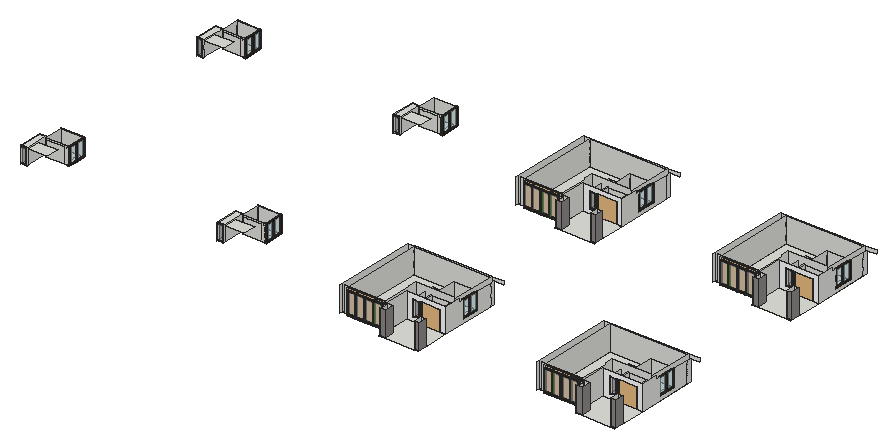
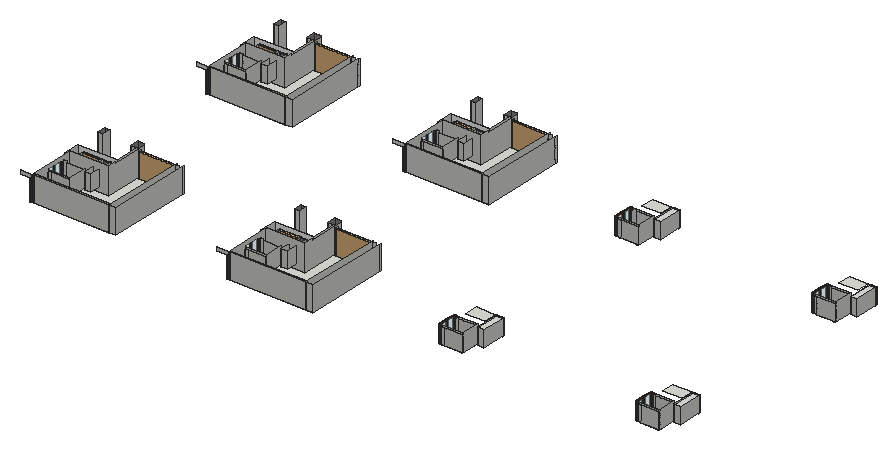
# SketchUp Ruby script. Lengths in inches.
U = 1.inch
M = Sketchup.active_model
def pt(a) = Geom::Point3d.new(a.map { |v| v * U })
def face(e, loops, mat)
  f = e.add_face(loops[0].map { |a| pt(a) })
  loops[1..].each { |l| e.add_face(l.map { |a| pt(a) }).erase! }
  f.material = f.back_material = mat if mat
  f
end
# faces: each face lists its corners as indices into pts; further lists are holes
def faces(e, pts, list, mat = nil) = list.each { |f| face(e, (f[0].is_a?(Array) ? f : [f]).map { |l| l.map { |i| pts[i] } }, mat) }
# xy, xz, yz: faces in a plane at the given z, y or x. An outline is a flat list of corners, or four numbers for a rectangle; further outlines are holes
def ring(l) = l.size == 4 ? [[l[0], l[1]], [l[2], l[1]], [l[2], l[3]], [l[0], l[3]]] : l.each_slice(2).to_a
def flat(e, list, mat, &to3) = list.each { |f| face(e, (f[0].is_a?(Array) ? f : [f]).map { |l| ring(l).map { |u, v| to3.(u, v) } }, mat) }
def xy(e, z, list, mat = nil) = flat(e, list, mat) { |x, y| [x, y, z] }
def xz(e, y, list, mat = nil) = flat(e, list, mat) { |x, z| [x, y, z] }
def yz(e, x, list, mat = nil) = flat(e, list, mat) { |y, z| [x, y, z] }
def lines(e, pts, list) = list.each { |a, b| e.add_line(pt(pts[a]), pt(pts[b])) }
# prism: a flat outline (further loops are holes) pulled along v
def prism(e, loops, v, mat = nil)
  f = face(e, loops, mat); d = Geom::Vector3d.new(v.map { |x| x * U })
  f.pushpull(f.normal.samedirection?(d) ? d.length : -d.length)
end
def box(e, o, s, mat = nil) = prism(e, [[o, [o[0] + s[0], o[1], o[2]], [o[0] + s[0], o[1] + s[1], o[2]], [o[0], o[1] + s[1], o[2]]]], [0, 0, s[2]], mat)
def at(x, y, z, deg = 0) = Geom::Transformation.translation(pt([x, y, z])) * Geom::Transformation.rotation(ORIGIN, Z_AXIS, deg.degrees)
def axes(o, x, y, z) = Geom::Transformation.new([*x, 0, *y, 0, *z, 0, *pt(o).to_a, 1])
def part(name) = M.definitions.add(name)
# library, detail: a bought-in or finely detailed component or shape, given as its bounding box
def library(name, o, s) = part(name).tap { |d| box(d.entities, o, s) }
def detail(e, o, s) = box(e.add_group.entities, o, s)
def put(e, d, t, mat = nil) = e.add_instance(d, t).tap { |i| i.material = mat if mat }
def group(e, t, mat = nil) = e.add_group.tap { |g| g.transformation = t; g.material = mat if mat }.entities
root = M.entities
M.materials.add("[Color M00]").color = [255, 255, 255]
M.materials.add("[Color M04]").color = [60, 133, 34]
M.materials.add("[Stone Marble]1").color = [143, 138, 136]
M.materials.add("[Translucent Glass Gray]1").color = [128, 128, 128]
M.materials["[Translucent Glass Gray]1"].alpha = 0.5
M.materials.add("[Translucent Glass Gray]2").color = [201, 201, 201]
M.materials["[Translucent Glass Gray]2"].alpha = 0.5
M.materials.add("[Translucent Glass Safety]").color = [204, 235, 244]
M.materials["[Translucent Glass Safety]"].alpha = 0.5
M.materials.add("[Wood Veneer 01]").color = [76, 44, 23]
M.materials.add("oak swatch").color = [40, 31, 19]
c1 = library("Curtains",[0,0,0],[121.73,8.19,117.22])
c2 = library("modern+door",[0,0,0],[59.06,11.8125,86.61])
c3 = part("Group\#6")
box(c3.entities,[0,0,0],[1.77,4.72,80.31],"oak swatch")
c4 = part("Exterior Sliding Doors")
xy(c4.entities,0,[[1.77,33.07,3.54,70.87],[1.77,70.87,3.54,108.66]])
xy(c4.entities,0,[[0,0,1.77,33.07],[0,108.66,1.77,141.73]],"oak swatch")
xy(c4.entities,4.72,[[0,4.72,1.77,33.07],[1.77,37.8,3.54,66.14],[1.77,75.88,3.54,103.9375],[0,108.66,1.77,137.01]],"oak swatch")
xy(c4.entities,75.59,[[1.77,37.8,3.54,66.14],[1.77,75.88,3.54,103.9375]])
xy(c4.entities,75.59,[[0,4.72,1.77,33.07],[0,108.66,1.77,137.01]],"oak swatch")
xy(c4.entities,80.31,[[0,0,1.77,33.07],[1.77,33.07,3.54,70.87],[1.77,70.87,3.54,108.66],[0,108.66,1.77,141.73]],"oak swatch")
xz(c4.entities,0,[[0,0,1.77,80.31]],"oak swatch")
xz(c4.entities,4.72,[[0,4.72,1.77,75.59]],"oak swatch")
xz(c4.entities,33.07,[[0,0,1.77,4.72],[1.77,0,3.54,80.31],[0,75.59,1.77,80.31]],"oak swatch")
xz(c4.entities,37.8,[[1.77,4.72,3.54,75.59]])
xz(c4.entities,66.14,[[1.77,4.72,3.54,75.59]],"oak swatch")
xz(c4.entities,70.87,[[1.77,0,3.54,80.31]])
xz(c4.entities,75.88,[[1.77,4.72,3.54,75.59]])
xz(c4.entities,103.9375,[[1.77,4.72,3.54,75.59]],"oak swatch")
xz(c4.entities,108.66,[[1.77,4.72,3.54,75.59]])
xz(c4.entities,108.66,[[0,0,3.54,4.72],[0,75.59,3.54,80.31]],"oak swatch")
xz(c4.entities,137.01,[[0,4.72,1.77,75.59]],"oak swatch")
xz(c4.entities,141.73,[[0,0,1.77,80.31]],"oak swatch")
yz(c4.entities,0,[[0,0,33.07,0,33.07,4.72,4.72,4.72,4.72,75.59,33.07,75.59,33.07,80.31,0,80.31],[108.66,0,141.73,0,141.73,80.31,108.66,80.31,108.66,75.59,137.01,75.59,137.01,4.72,108.66,4.72]],"oak swatch")
yz(c4.entities,1.77,[[4.72,4.72,33.07,75.59],[37.8,4.72,66.14,75.59],[75.88,4.72,103.9375,75.59],[108.66,4.72,137.01,75.59]],"[Translucent Glass Gray]2")
yz(c4.entities,1.77,[[0,0,33.07,0,33.07,4.72,4.72,4.72,4.72,75.59,33.07,75.59,33.07,80.31,0,80.31],[[33.07,0,70.87,80.31],[37.8,4.72,66.14,75.59]],[[70.87,0,141.73,80.31],[108.66,4.72,137.01,75.59],[75.88,4.72,103.9375,75.59]]],"oak swatch")
yz(c4.entities,3.54,[[[33.07,0,70.87,80.31],[37.8,4.72,66.14,75.59]],[[70.87,0,108.66,80.31],[75.88,4.72,103.9375,75.59]]],"oak swatch")
put(c4.entities,c3,at(0,33.07,0))
put(c4.entities,c3,at(0,103.9375,0))
c5 = part("Group\#4")
g1 = group(c5.entities,at(0,0,0))
xy(g1,0,[[0,0,6,48]],"[Wood Veneer 01]")
xy(g1,4,[[0,4,1.8125,44],[1.8125,4,6,44]])
xy(g1,80,[[0,4,1.8125,44],[1.8125,4,6,44]])
xy(g1,84,[[0,0,6,48]],"[Wood Veneer 01]")
xz(g1,0,[[0,0,6,84]],"[Wood Veneer 01]")
xz(g1,4,[[0,4,1.8125,80],[1.8125,4,6,80]])
xz(g1,44,[[0,4,1.8125,80],[1.8125,4,6,80]])
xz(g1,48,[[0,0,6,84]],"[Wood Veneer 01]")
yz(g1,0,[[[0,0,48,84],[4,4,44,80]]],"[Wood Veneer 01]")
yz(g1,1.8125,[[4,4,44,80]],"[Translucent Glass Safety]")
yz(g1,6,[[[0,0,48,84],[4,4,44,80]]],"oak swatch")
g2 = group(c5.entities,at(0,48,0),"oak swatch")
xy(g2,0,[[0,0,6,48]],"[Wood Veneer 01]")
xy(g2,4,[[0,4,1.8125,44],[1.8125,4,6,44]])
xy(g2,80,[[0,4,1.8125,44],[1.8125,4,6,44]])
xy(g2,84,[[0,0,6,48]],"[Wood Veneer 01]")
xz(g2,0,[[0,0,6,84]],"[Wood Veneer 01]")
xz(g2,4,[[0,4,1.8125,80],[1.8125,4,6,80]])
xz(g2,44,[[0,4,1.8125,80],[1.8125,4,6,80]])
xz(g2,48,[[0,0,6,84]],"[Wood Veneer 01]")
yz(g2,0,[[[0,0,48,84],[4,4,44,80]]],"[Wood Veneer 01]")
yz(g2,1.8125,[[4,4,44,80]],"[Translucent Glass Safety]")
yz(g2,6,[[[0,0,48,84],[4,4,44,80]]],"oak swatch")
c6 = part("Group\#71")
prism(c6.entities,[[[0,0.79,82.68],[13.78,0.79,82.68],[13.78,0.79,0],[0,0.79,0]],[[1.97,0.79,80.71],[1.97,0.79,1.97],[11.8125,0.79,1.97],[11.8125,0.79,80.71]]],[0,-3.54,0])
xy(root,6,[[2276.89,590.5625,2304.32,595.6875],[2304.32,590.5625,2435.04,590.5625,2435.04,633.25,2456.54,633.25,2456.54,747.5625,2430.86,747.5625,2430.86,806.0625,2346.59,806.0625,2346.59,747.5625,2276.89,747.5625,2276.89,636.625,2304.32,636.625],[2435.04,590.5625,2456.54,595.6875],[3169.48,590.5625,3196.91,595.6875],[3196.91,590.5625,3327.63,590.5625,3327.63,633.25,3349.13,633.25,3349.13,747.5625,3323.45,747.5625,3323.45,806.0625,3239.18,806.0625,3239.18,747.5625,3169.48,747.5625,3169.48,636.625,3196.91,636.625],
  [3327.63,590.5625,3349.13,595.6875],[2276.89,595.6875,2304.32,636.625],[2435.04,595.6875,2456.54,633.25],[3169.48,595.6875,3196.91,636.625],[3327.63,595.6875,3349.13,633.25],
  [2097.23,636.6875,2258.0625,645.91],[2258.0625,636.6875,2276.89,645.91],[2989.82,636.6875,3150.65,645.91],[3150.65,636.6875,3169.48,645.91],[2064.92,645.91,2097.23,1019],
  [2097.23,645.91,2266.54,645.91,2266.54,811.54,2447.32,811.54,2447.32,1019,2440.84,1019,2440.84,1011.63,2097.23,1011.63],[2266.54,645.91,2276.89,645.91,2276.89,747.5625,2346.59,747.5625,2346.59,806.0625,2430.86,806.0625,2430.86,747.5625,2447.32,747.5625,2447.32,811.54,2266.54,811.54],[2957.51,645.91,2989.82,1019],[2989.82,645.91,3159.13,645.91,3159.13,811.54,3339.91,811.54,3339.91,1019,3333.43,1019,3333.43,1011.63,2989.82,1011.63],[3159.13,645.91,3169.48,645.91,3169.48,747.5625,3239.18,747.5625,3239.18,806.0625,3323.45,806.0625,3323.45,747.5625,3339.91,747.5625,3339.91,811.54,3159.13,811.54],
  [2447.32,747.5625,2456.54,1019],[3339.91,747.5625,3349.13,1019],[2097.23,1011.63,2440.84,1019],[2989.82,1011.63,3333.43,1019],[2276.89,1589.92,2304.32,1595.04],
  [2304.32,1589.92,2435.04,1589.92,2435.04,1632.6,2456.54,1632.6,2456.54,1746.92,2430.86,1746.92,2430.86,1805.42,2346.59,1805.42,2346.59,1746.92,2276.89,1746.92,2276.89,1635.98,2304.32,1635.98],[2435.04,1589.92,2456.54,1595.04],[3169.48,1589.92,3196.91,1595.04],[3196.91,1589.92,3327.63,1589.92,3327.63,1632.6,3349.13,1632.6,3349.13,1746.92,3323.45,1746.92,3323.45,1805.42,3239.18,1805.42,3239.18,1746.92,3169.48,1746.92,3169.48,1635.98,3196.91,1635.98],[3327.63,1589.92,3349.13,1595.04],
  [2276.89,1595.04,2304.32,1635.98],[2435.04,1595.04,2456.54,1632.6],[3169.48,1595.04,3196.91,1635.98],[3327.63,1595.04,3349.13,1632.6],[2097.23,1636.04,2258.0625,1645.27],
  [2258.0625,1636.04,2276.89,1645.27],[2989.82,1636.04,3150.65,1645.27],[3150.65,1636.04,3169.48,1645.27],[2064.92,1645.27,2097.23,2018.36],[2097.23,1645.27,2266.54,1645.27,2266.54,1810.9,2447.32,1810.9,2447.32,2018.36,2440.84,2018.36,2440.84,2010.98,2097.23,2010.98],
  [2266.54,1645.27,2276.89,1645.27,2276.89,1746.92,2346.59,1746.92,2346.59,1805.42,2430.86,1805.42,2430.86,1746.92,2447.32,1746.92,2447.32,1810.9,2266.54,1810.9],[2957.51,1645.27,2989.82,2018.36],[2989.82,1645.27,3159.13,1645.27,3159.13,1810.9,3339.91,1810.9,3339.91,2018.36,3333.43,2018.36,3333.43,2010.98,2989.82,2010.98],[3159.13,1645.27,3169.48,1645.27,3169.48,1746.92,3239.18,1746.92,3239.18,1805.42,3323.45,1805.42,3323.45,1746.92,3339.91,1746.92,3339.91,1810.9,3159.13,1810.9],[2447.32,1746.92,2456.54,2018.36],
  [3339.91,1746.92,3349.13,2018.36],[2097.23,2010.98,2440.84,2018.36],[2989.82,2010.98,3333.43,2018.36]])
xy(root,18.5,[[563.18,847.15,645.68,931.09],[645.68,847.15,662.14,931.09],[662.14,847.15,671.36,931.78],[1455.77,847.15,1538.27,931.09],[1538.27,847.15,1554.73,931.09],
  [1554.73,847.15,1563.95,931.78],[563.18,931.09,645.68,931.22],[645.68,931.09,662.14,931.22],[1455.77,931.09,1538.27,931.22],[1538.27,931.09,1554.73,931.22],
  [563.18,931.22,645.68,931.78],[645.68,931.22,662.14,931.78],[1455.77,931.22,1538.27,931.78],[1538.27,931.22,1554.73,931.78],[563.18,1846.51,645.68,1930.45],
  [645.68,1846.51,662.14,1930.45],[662.14,1846.51,671.36,1931.13],[1455.77,1846.51,1538.27,1930.45],[1538.27,1846.51,1554.73,1930.45],[1554.73,1846.51,1563.95,1931.13],
  [563.18,1930.45,645.68,1930.57],[645.68,1930.45,662.14,1930.57],[1455.77,1930.45,1538.27,1930.57],[1538.27,1930.45,1554.73,1930.57],[563.18,1930.57,645.68,1931.13],
  [645.68,1930.57,662.14,1931.13],[1455.77,1930.57,1538.27,1931.13],[1538.27,1930.57,1554.73,1931.13]])
xy(root,21.58,[[523.18,749.87,552.96,755.77],[1415.77,749.87,1445.55,755.77],[523.18,1749.22,552.96,1755.13],[1415.77,1749.22,1445.55,1755.13]])
xy(root,23.1875,[[2348.36,844.85,2430.86,928.79],[2430.86,844.85,2447.32,928.79],[2447.32,844.85,2456.54,929.47],[3240.94,844.85,3323.45,928.79],[3323.45,844.85,3339.91,928.79],
  [3339.91,844.85,3349.13,929.47],[2348.36,928.79,2430.86,928.91],[2430.86,928.79,2447.32,928.91],[3240.94,928.79,3323.45,928.91],[3323.45,928.79,3339.91,928.91],
  [2348.36,928.91,2430.86,929.47],[2430.86,928.91,2447.32,929.47],[3240.94,928.91,3323.45,929.47],[3323.45,928.91,3339.91,929.47],[2348.36,1844.2,2430.86,1928.14],
  [2430.86,1844.2,2447.32,1928.14],[2447.32,1844.2,2456.54,1928.83],[3240.94,1844.2,3323.45,1928.14],[3323.45,1844.2,3339.91,1928.14],[3339.91,1844.2,3349.13,1928.83],
  [2348.36,1928.14,2430.86,1928.27],[2430.86,1928.14,2447.32,1928.27],[3240.94,1928.14,3323.45,1928.27],[3323.45,1928.14,3339.91,1928.27],[2348.36,1928.27,2430.86,1928.83],
  [2430.86,1928.27,2447.32,1928.83],[3240.94,1928.27,3323.45,1928.83],[3323.45,1928.27,3339.91,1928.83]])
xy(root,26.27,[[2308.36,747.5625,2338.14,753.47],[3200.95,747.5625,3230.73,753.47],[2308.36,1746.92,2338.14,1752.82],[3200.95,1746.92,3230.73,1752.82]])
xy(root,89.1875,[[656.89,931.47,657.58,931.78],[1549.48,931.47,1550.17,931.78],[656.89,1930.82,657.58,1931.13],[1549.48,1930.82,1550.17,1931.13]])
xy(root,93.27,[[561.42,749.87,645.68,808.37],[1454.01,749.87,1538.27,808.37],[561.42,1749.22,645.68,1807.72],[1454.01,1749.22,1538.27,1807.72]])
xy(root,93.3,[[523.18,749.87,552.96,755.77],[1415.77,749.87,1445.55,755.77],[523.18,1749.22,552.96,1755.13],[1415.77,1749.22,1445.55,1755.13]],"[Wood Veneer 01]")
xz(root,595.6875,[[2276.89,6,2304.32,118.5],[2435.04,6,2456.54,118.5],[3169.48,6,3196.91,118.5],[3327.63,6,3349.13,118.5]],"[Stone Marble]1")
xz(root,633.25,[[2435.04,6,2456.54,118.5],[3327.63,6,3349.13,118.5]])
xz(root,636.625,[[2276.89,6,2304.32,118.5],[3169.48,6,3196.91,118.5]])
xz(root,636.6875,[[2258.0625,6,2276.89,109.625],[3150.65,6,3169.48,109.625]])
xz(root,645.91,[[2079.67,6,2097.23,118.5],[2258.0625,6,2266.54,118.5],[2972.26,6,2989.82,118.5],[3150.65,6,3159.13,118.5]])
xz(root,747.5625,[[[2276.89,6,2346.59,6,2346.59,97.96,2430.86,97.96,2430.86,6,2456.54,6,2456.54,118.5,2276.89,118.5],[2308.36,26.27,2338.14,97.99]],[[3169.48,6,3239.18,6,3239.18,97.96,3323.45,97.96,3323.45,6,3349.13,6,3349.13,118.5,3169.48,118.5],[3200.95,26.27,3230.73,97.99]]],"[Color M00]")
xz(root,750.52,[[2311.9,27.4375,2334.6,95.26],[3204.49,27.4375,3227.19,95.26]],"[Translucent Glass Gray]1")
xz(root,752.82,[[526.72,22.75,549.42,90.57],[1419.31,22.75,1442.01,90.57]],"[Translucent Glass Gray]1")
xz(root,806.0625,[[2346.59,6,2430.86,97.96],[3239.18,6,3323.45,97.96]])
xz(root,811.54,[[2266.54,6,2266.54,126,2440.84,126,2440.84,118.5,2447.32,118.5,2447.32,6],[3159.13,6,3159.13,126,3333.43,126,3333.43,118.5,3339.91,118.5,3339.91,6]])
xz(root,844.85,[[2348.36,23.1875,2430.86,93.875],[2430.86,23.1875,2430.86,101.6875,2442.07,101.6875,2442.07,93.875,2447.32,93.875,2447.32,23.1875],[2447.32,23.1875,2456.54,102.625],[3240.94,23.1875,3323.45,93.875],[3323.45,23.1875,3323.45,101.6875,3334.66,101.6875,3334.66,93.875,3339.91,93.875,3339.91,23.1875],
  [3339.91,23.1875,3349.13,102.625]])
xz(root,847.15,[[563.18,18.5,645.68,89.1875],[645.68,18.5,645.68,97,656.89,97,656.89,89.1875,662.14,89.1875,662.14,18.5],[662.14,18.5,671.36,97.9375],[1455.77,18.5,1538.27,89.1875],[1538.27,18.5,1538.27,97,1549.48,97,1549.48,89.1875,1554.73,89.1875,1554.73,18.5],
  [1554.73,18.5,1563.95,97.9375],[563.18,89.1875,645.68,97],[656.89,89.1875,657.58,97],[657.58,89.1875,662.14,89.1875,662.14,97.9375,658.26,97.9375,658.26,97.25,657.58,97.25],[1455.77,89.1875,1538.27,97],
  [1549.48,89.1875,1550.17,97],[1550.17,89.1875,1554.73,89.1875,1554.73,97.9375,1550.85,97.9375,1550.85,97.25,1550.17,97.25]])
xz(root,857.25,[[2307.7,25.52,2338.14,97.96],[3200.29,25.52,3230.73,97.96]])
xz(root,859.56,[[522.52,20.84,552.96,93.27],[1415.11,20.84,1445.55,93.27]])
xz(root,928.79,[[2348.36,23.1875,2447.32,23.1875,2447.32,102.625,2443.44,102.625,2443.44,101.9375,2442.07,101.9375,2442.07,101.6875,2348.36,101.6875],[3240.94,23.1875,3339.91,23.1875,3339.91,102.625,3336.03,102.625,3336.03,101.9375,3334.66,101.9375,3334.66,101.6875,3240.94,101.6875]])
xz(root,928.91,[[2348.36,23.1875,2348.36,101.6875,2442.07,101.6875,2442.07,93.875,2442.76,93.875,2442.76,101.9375,2443.44,101.9375,2443.44,102.625,2447.32,102.625,2447.32,23.1875],[3240.94,23.1875,3240.94,101.6875,3334.66,101.6875,3334.66,93.875,3335.34,93.875,3335.34,101.9375,3336.03,101.9375,3336.03,102.625,3339.91,102.625,3339.91,23.1875]])
xz(root,929.47,[[2348.36,23.1875,2430.86,93.875],[2430.86,23.1875,2447.32,93.875],[2447.32,23.1875,2456.54,102.625],[3240.94,23.1875,3323.45,93.875],[3323.45,23.1875,3339.91,93.875],
  [3339.91,23.1875,3349.13,102.625]])
xz(root,931.09,[[563.18,18.5,662.14,18.5,662.14,97.9375,658.26,97.9375,658.26,97.25,656.89,97.25,656.89,97,563.18,97],[1455.77,18.5,1554.73,18.5,1554.73,97.9375,1550.85,97.9375,1550.85,97.25,1549.48,97.25,1549.48,97,1455.77,97]])
xz(root,931.22,[[563.18,18.5,563.18,97,656.89,97,656.89,89.1875,657.58,89.1875,657.58,97.25,658.26,97.25,658.26,97.9375,662.14,97.9375,662.14,18.5],[1455.77,18.5,1455.77,97,1549.48,97,1549.48,89.1875,1550.17,89.1875,1550.17,97.25,1550.85,97.25,1550.85,97.9375,1554.73,97.9375,1554.73,18.5]])
xz(root,931.47,[[656.89,89.1875,657.58,97.25],[1549.48,89.1875,1550.17,97.25]])
xz(root,931.78,[[563.18,18.5,645.68,89.1875],[645.68,18.5,662.14,89.1875],[662.14,18.5,671.36,97.9375],[1455.77,18.5,1538.27,89.1875],[1538.27,18.5,1554.73,89.1875],
  [1554.73,18.5,1563.95,97.9375],[563.18,89.1875,656.89,97.9375],[656.89,89.1875,657.58,97.9375],[657.58,89.1875,662.14,97.9375],[1455.77,89.1875,1549.48,97.9375],
  [1549.48,89.1875,1550.17,97.9375],[1550.17,89.1875,1554.73,97.9375]])
xz(root,1011.63,[[2097.23,6,2440.84,118.5],[2989.82,6,3333.43,118.5]])
xz(root,1019,[[2064.92,6,2097.23,118.5],[2097.23,6,2440.84,118.5],[2440.84,6,2447.32,118.5],[2447.32,6,2447.32,118.5,2500.29,118.5,2500.29,102.625,2456.54,102.625,2456.54,6],[2957.51,6,2989.82,118.5],
  [2989.82,6,3333.43,118.5],[3333.43,6,3339.91,118.5],[3339.91,6,3339.91,118.5,3392.88,118.5,3392.88,102.625,3349.13,102.625,3349.13,6]])
xz(root,1595.04,[[2276.89,6,2304.32,118.5],[2435.04,6,2456.54,118.5],[3169.48,6,3196.91,118.5],[3327.63,6,3349.13,118.5]],"[Stone Marble]1")
xz(root,1632.6,[[2435.04,6,2456.54,118.5],[3327.63,6,3349.13,118.5]])
xz(root,1635.98,[[2276.89,6,2304.32,118.5],[3169.48,6,3196.91,118.5]])
xz(root,1636.04,[[2258.0625,6,2276.89,109.625],[3150.65,6,3169.48,109.625]])
xz(root,1645.27,[[2079.67,6,2097.23,118.5],[2258.0625,6,2266.54,118.5],[2972.26,6,2989.82,118.5],[3150.65,6,3159.13,118.5]])
xz(root,1746.92,[[[2276.89,6,2346.59,6,2346.59,97.96,2430.86,97.96,2430.86,6,2456.54,6,2456.54,118.5,2276.89,118.5],[2308.36,26.27,2338.14,97.99]],[[3169.48,6,3239.18,6,3239.18,97.96,3323.45,97.96,3323.45,6,3349.13,6,3349.13,118.5,3169.48,118.5],[3200.95,26.27,3230.73,97.99]]],"[Color M00]")
xz(root,1749.87,[[2311.9,27.4375,2334.6,95.26],[3204.49,27.4375,3227.19,95.26]],"[Translucent Glass Gray]1")
xz(root,1752.18,[[526.72,22.75,549.42,90.57],[1419.31,22.75,1442.01,90.57]],"[Translucent Glass Gray]1")
xz(root,1805.42,[[2346.59,6,2430.86,97.96],[3239.18,6,3323.45,97.96]])
xz(root,1810.9,[[2266.54,6,2266.54,126,2440.84,126,2440.84,118.5,2447.32,118.5,2447.32,6],[3159.13,6,3159.13,126,3333.43,126,3333.43,118.5,3339.91,118.5,3339.91,6]])
xz(root,1844.2,[[2348.36,23.1875,2430.86,93.875],[2430.86,23.1875,2430.86,101.6875,2442.07,101.6875,2442.07,93.875,2447.32,93.875,2447.32,23.1875],[2447.32,23.1875,2456.54,102.625],[3240.94,23.1875,3323.45,93.875],[3323.45,23.1875,3323.45,101.6875,3334.66,101.6875,3334.66,93.875,3339.91,93.875,3339.91,23.1875],
  [3339.91,23.1875,3349.13,102.625]])
xz(root,1846.51,[[563.18,18.5,645.68,89.1875],[645.68,18.5,645.68,97,656.89,97,656.89,89.1875,662.14,89.1875,662.14,18.5],[662.14,18.5,671.36,97.9375],[1455.77,18.5,1538.27,89.1875],[1538.27,18.5,1538.27,97,1549.48,97,1549.48,89.1875,1554.73,89.1875,1554.73,18.5],
  [1554.73,18.5,1563.95,97.9375],[563.18,89.1875,645.68,97],[656.89,89.1875,657.58,97],[657.58,89.1875,662.14,89.1875,662.14,97.9375,658.26,97.9375,658.26,97.25,657.58,97.25],[1455.77,89.1875,1538.27,97],
  [1549.48,89.1875,1550.17,97],[1550.17,89.1875,1554.73,89.1875,1554.73,97.9375,1550.85,97.9375,1550.85,97.25,1550.17,97.25]])
xz(root,1856.6,[[2307.7,25.52,2338.14,97.96],[3200.29,25.52,3230.73,97.96]])
xz(root,1858.91,[[522.52,20.84,552.96,93.27],[1415.11,20.84,1445.55,93.27]])
xz(root,1928.14,[[2348.36,23.1875,2447.32,23.1875,2447.32,102.625,2443.44,102.625,2443.44,101.9375,2442.07,101.9375,2442.07,101.6875,2348.36,101.6875],[3240.94,23.1875,3339.91,23.1875,3339.91,102.625,3336.03,102.625,3336.03,101.9375,3334.66,101.9375,3334.66,101.6875,3240.94,101.6875]])
xz(root,1928.27,[[2348.36,23.1875,2348.36,101.6875,2442.07,101.6875,2442.07,93.875,2442.76,93.875,2442.76,101.9375,2443.44,101.9375,2443.44,102.625,2447.32,102.625,2447.32,23.1875],[3240.94,23.1875,3240.94,101.6875,3334.66,101.6875,3334.66,93.875,3335.34,93.875,3335.34,101.9375,3336.03,101.9375,3336.03,102.625,3339.91,102.625,3339.91,23.1875]])
xz(root,1928.83,[[2348.36,23.1875,2430.86,93.875],[2430.86,23.1875,2447.32,93.875],[2447.32,23.1875,2456.54,102.625],[3240.94,23.1875,3323.45,93.875],[3323.45,23.1875,3339.91,93.875],
  [3339.91,23.1875,3349.13,102.625]])
xz(root,1930.45,[[563.18,18.5,662.14,18.5,662.14,97.9375,658.26,97.9375,658.26,97.25,656.89,97.25,656.89,97,563.18,97],[1455.77,18.5,1554.73,18.5,1554.73,97.9375,1550.85,97.9375,1550.85,97.25,1549.48,97.25,1549.48,97,1455.77,97]])
xz(root,1930.57,[[563.18,18.5,563.18,97,656.89,97,656.89,89.1875,657.58,89.1875,657.58,97.25,658.26,97.25,658.26,97.9375,662.14,97.9375,662.14,18.5],[1455.77,18.5,1455.77,97,1549.48,97,1549.48,89.1875,1550.17,89.1875,1550.17,97.25,1550.85,97.25,1550.85,97.9375,1554.73,97.9375,1554.73,18.5]])
xz(root,1930.82,[[656.89,89.1875,657.58,97.25],[1549.48,89.1875,1550.17,97.25]])
xz(root,1931.13,[[563.18,18.5,645.68,89.1875],[645.68,18.5,662.14,89.1875],[662.14,18.5,671.36,97.9375],[1455.77,18.5,1538.27,89.1875],[1538.27,18.5,1554.73,89.1875],
  [1554.73,18.5,1563.95,97.9375],[563.18,89.1875,656.89,97.9375],[656.89,89.1875,657.58,97.9375],[657.58,89.1875,662.14,97.9375],[1455.77,89.1875,1549.48,97.9375],
  [1549.48,89.1875,1550.17,97.9375],[1550.17,89.1875,1554.73,97.9375]])
xz(root,2010.98,[[2097.23,6,2440.84,118.5],[2989.82,6,3333.43,118.5]])
xz(root,2018.36,[[2064.92,6,2097.23,118.5],[2097.23,6,2440.84,118.5],[2440.84,6,2447.32,118.5],[2447.32,6,2447.32,118.5,2500.29,118.5,2500.29,102.625,2456.54,102.625,2456.54,6],[2957.51,6,2989.82,118.5],
  [2989.82,6,3333.43,118.5],[3333.43,6,3339.91,118.5],[3339.91,6,3339.91,118.5,3392.88,118.5,3392.88,102.625,3349.13,102.625,3349.13,6]])
yz(root,523.18,[[749.87,20.02,755.77,21.58],[1749.22,20.02,1755.13,21.58],[749.87,21.58,755.77,93.3],[1749.22,21.58,1755.13,93.3]],"[Wood Veneer 01]")
yz(root,552.96,[[859.56,20.84,755.77,21.58,755.77,93.3,859.56,93.27],[1858.91,20.84,1755.13,21.58,1755.13,93.3,1858.91,93.27],[749.87,21.58,755.77,93.3],[1749.22,21.58,1755.13,93.3]])
yz(root,563.18,[[847.15,18.5,931.09,97],[931.09,18.5,931.22,89.1875],[931.22,18.5,931.78,89.1875],[1846.51,18.5,1930.45,97],[1930.45,18.5,1930.57,89.1875],
  [1930.57,18.5,1931.13,89.1875],[931.09,89.1875,931.22,97],[931.22,89.1875,931.78,89.1875,931.78,97.9375,931.09,97.9375,931.09,97,931.22,97],[1930.45,89.1875,1930.57,97],[1930.57,89.1875,1931.13,89.1875,1931.13,97.9375,1930.45,97.9375,1930.45,97,1930.57,97]])
yz(root,656.89,[[931.47,89.1875,931.47,97.25,931.09,97.25,931.09,97.9375,931.78,97.9375,931.78,89.1875],[1930.82,89.1875,1930.82,97.25,1930.45,97.25,1930.45,97.9375,1931.13,97.9375,1931.13,89.1875]])
yz(root,657.58,[[931.47,89.1875,931.47,97.25,931.09,97.25,931.09,97.9375,931.78,97.9375,931.78,89.1875],[931.22,89.1875,931.47,97.25],[1930.82,89.1875,1930.82,97.25,1930.45,97.25,1930.45,97.9375,1931.13,97.9375,1931.13,89.1875],[1930.57,89.1875,1930.82,97.25]])
yz(root,662.14,[[931.09,18.5,931.22,89.1875],[931.22,18.5,931.78,89.1875],[1930.45,18.5,1930.57,89.1875],[1930.57,18.5,1931.13,89.1875],[931.09,89.1875,931.22,97.9375],
  [931.22,89.1875,931.78,97.9375],[1930.45,89.1875,1930.57,97.9375],[1930.57,89.1875,1931.13,97.9375]])
yz(root,1415.77,[[749.87,20.02,755.77,21.58],[1749.22,20.02,1755.13,21.58],[749.87,21.58,755.77,93.3],[1749.22,21.58,1755.13,93.3]],"[Wood Veneer 01]")
yz(root,1445.55,[[859.56,20.84,755.77,21.58,755.77,93.3,859.56,93.27],[1858.91,20.84,1755.13,21.58,1755.13,93.3,1858.91,93.27],[749.87,21.58,755.77,93.3],[1749.22,21.58,1755.13,93.3]])
yz(root,1455.77,[[847.15,18.5,931.09,97],[931.09,18.5,931.22,89.1875],[931.22,18.5,931.78,89.1875],[1846.51,18.5,1930.45,97],[1930.45,18.5,1930.57,89.1875],
  [1930.57,18.5,1931.13,89.1875],[931.09,89.1875,931.22,97],[931.22,89.1875,931.78,89.1875,931.78,97.9375,931.09,97.9375,931.09,97,931.22,97],[1930.45,89.1875,1930.57,97],[1930.57,89.1875,1931.13,89.1875,1931.13,97.9375,1930.45,97.9375,1930.45,97,1930.57,97]])
yz(root,1549.48,[[931.47,89.1875,931.47,97.25,931.09,97.25,931.09,97.9375,931.78,97.9375,931.78,89.1875],[1930.82,89.1875,1930.82,97.25,1930.45,97.25,1930.45,97.9375,1931.13,97.9375,1931.13,89.1875]])
yz(root,1550.17,[[931.47,89.1875,931.47,97.25,931.09,97.25,931.09,97.9375,931.78,97.9375,931.78,89.1875],[931.22,89.1875,931.47,97.25],[1930.82,89.1875,1930.82,97.25,1930.45,97.25,1930.45,97.9375,1931.13,97.9375,1931.13,89.1875],[1930.57,89.1875,1930.82,97.25]])
yz(root,1554.73,[[931.09,18.5,931.22,89.1875],[931.22,18.5,931.78,89.1875],[1930.45,18.5,1930.57,89.1875],[1930.57,18.5,1931.13,89.1875],[931.09,89.1875,931.22,97.9375],
  [931.22,89.1875,931.78,97.9375],[1930.45,89.1875,1930.57,97.9375],[1930.57,89.1875,1931.13,97.9375]])
yz(root,2064.92,[[636.6875,6,645.91,118.5],[645.91,6,1019,118.5],[1636.04,6,1645.27,118.5],[1645.27,6,2018.36,118.5]])
yz(root,2097.23,[[636.6875,6,645.91,118.5],[645.91,6,1011.63,118.5],[1011.63,6,1019,118.5],[1636.04,6,1645.27,118.5],[1645.27,6,2010.98,118.5],
  [2010.98,6,2018.36,118.5]])
yz(root,2258.0625,[[636.6875,6,645.91,118.5],[1636.04,6,1645.27,118.5]])
yz(root,2266.54,[[645.91,6,645.91,118.5,774.3125,118.5,774.3125,126,811.54,126,811.54,6],[1645.27,6,1645.27,118.5,1773.67,118.5,1773.67,126,1810.9,126,1810.9,6]])
yz(root,2276.89,[[595.6875,6,636.625,109.625],[636.6875,6,747.5625,118.5],[1595.04,6,1635.98,109.625],[1636.04,6,1746.92,118.5]])
yz(root,2304.32,[[595.6875,6,636.625,118.5],[1595.04,6,1635.98,118.5]],"[Stone Marble]1")
yz(root,2308.36,[[747.5625,24.71,753.47,26.27],[1746.92,24.71,1752.82,26.27],[747.5625,26.27,753.47,97.99],[1746.92,26.27,1752.82,97.99]],"[Wood Veneer 01]")
yz(root,2338.14,[[857.25,25.52,753.47,26.27,753.47,97.99,857.25,97.96],[1856.6,25.52,1752.82,26.27,1752.82,97.99,1856.6,97.96],[747.5625,26.27,753.47,97.99],[1746.92,26.27,1752.82,97.99]])
yz(root,2346.59,[[747.5625,6,806.0625,97.96],[1746.92,6,1805.42,97.96]])
yz(root,2348.36,[[844.85,23.1875,928.79,101.6875],[928.79,23.1875,928.91,93.875],[928.91,23.1875,929.47,93.875],[1844.2,23.1875,1928.14,101.6875],[1928.14,23.1875,1928.27,93.875],
  [1928.27,23.1875,1928.83,93.875]])
yz(root,2430.86,[[747.5625,6,806.0625,97.96],[1746.92,6,1805.42,97.96]])
yz(root,2435.04,[[595.6875,6,633.25,118.5],[1595.04,6,1632.6,118.5]])
yz(root,2440.84,[[1011.63,6,1019,118.5],[2010.98,6,2018.36,118.5]])
yz(root,2447.32,[[[811.54,6,1019,118.5],[844.85,23.1875,929.47,102.625]],[[1810.9,6,2018.36,118.5],[1844.2,23.1875,1928.83,102.625]],[928.79,23.1875,928.91,93.875],[928.91,23.1875,929.47,93.875],[1928.14,23.1875,1928.27,93.875],
  [1928.27,23.1875,1928.83,93.875]])
yz(root,2456.54,[[747.5625,6,999.35,6,999.35,102.625,929.47,102.625,929.47,23.1875,844.85,23.1875,844.85,102.625,822.54,102.625,822.54,118.5,747.5625,118.5],[999.35,6,1019,102.625],[1746.92,6,1998.71,6,1998.71,102.625,1928.83,102.625,1928.83,23.1875,1844.2,23.1875,1844.2,102.625,1821.9,102.625,1821.9,118.5,1746.92,118.5],[1998.71,6,2018.36,102.625]])
yz(root,2456.54,[[595.6875,6,633.25,118.5],[1595.04,6,1632.6,118.5]],"[Stone Marble]1")
yz(root,2957.51,[[636.6875,6,645.91,118.5],[645.91,6,1019,118.5],[1636.04,6,1645.27,118.5],[1645.27,6,2018.36,118.5]])
yz(root,2989.82,[[636.6875,6,645.91,118.5],[645.91,6,1011.63,118.5],[1011.63,6,1019,118.5],[1636.04,6,1645.27,118.5],[1645.27,6,2010.98,118.5],
  [2010.98,6,2018.36,118.5]])
yz(root,3150.65,[[636.6875,6,645.91,118.5],[1636.04,6,1645.27,118.5]])
yz(root,3159.13,[[645.91,6,645.91,118.5,774.3125,118.5,774.3125,126,811.54,126,811.54,6],[1645.27,6,1645.27,118.5,1773.67,118.5,1773.67,126,1810.9,126,1810.9,6]])
yz(root,3169.48,[[595.6875,6,636.625,109.625],[636.6875,6,747.5625,118.5],[1595.04,6,1635.98,109.625],[1636.04,6,1746.92,118.5]])
yz(root,3196.91,[[595.6875,6,636.625,118.5],[1595.04,6,1635.98,118.5]],"[Stone Marble]1")
yz(root,3200.95,[[747.5625,24.71,753.47,26.27],[1746.92,24.71,1752.82,26.27],[747.5625,26.27,753.47,97.99],[1746.92,26.27,1752.82,97.99]],"[Wood Veneer 01]")
yz(root,3230.73,[[857.25,25.52,753.47,26.27,753.47,97.99,857.25,97.96],[1856.6,25.52,1752.82,26.27,1752.82,97.99,1856.6,97.96],[747.5625,26.27,753.47,97.99],[1746.92,26.27,1752.82,97.99]])
yz(root,3239.18,[[747.5625,6,806.0625,97.96],[1746.92,6,1805.42,97.96]])
yz(root,3240.94,[[844.85,23.1875,928.79,101.6875],[928.79,23.1875,928.91,93.875],[928.91,23.1875,929.47,93.875],[1844.2,23.1875,1928.14,101.6875],[1928.14,23.1875,1928.27,93.875],
  [1928.27,23.1875,1928.83,93.875]])
yz(root,3323.45,[[747.5625,6,806.0625,97.96],[1746.92,6,1805.42,97.96]])
yz(root,3327.63,[[595.6875,6,633.25,118.5],[1595.04,6,1632.6,118.5]])
yz(root,3333.43,[[1011.63,6,1019,118.5],[2010.98,6,2018.36,118.5]])
yz(root,3339.91,[[[811.54,6,1019,118.5],[844.85,23.1875,929.47,102.625]],[[1810.9,6,2018.36,118.5],[1844.2,23.1875,1928.83,102.625]],[928.79,23.1875,928.91,93.875],[928.91,23.1875,929.47,93.875],[1928.14,23.1875,1928.27,93.875],
  [1928.27,23.1875,1928.83,93.875]])
yz(root,3349.13,[[747.5625,6,999.35,6,999.35,102.625,929.47,102.625,929.47,23.1875,844.85,23.1875,844.85,102.625,822.54,102.625,822.54,118.5,747.5625,118.5],[999.35,6,1019,102.625],[1746.92,6,1998.71,6,1998.71,102.625,1928.83,102.625,1928.83,23.1875,1844.2,23.1875,1844.2,102.625,1821.9,102.625,1821.9,118.5,1746.92,118.5],[1998.71,6,2018.36,102.625]])
yz(root,3349.13,[[595.6875,6,633.25,118.5],[1595.04,6,1632.6,118.5]],"[Stone Marble]1")
p = [[523.18,755.77,21.58],[522.52,859.56,20.84],[522.52,859.56,93.27],[523.18,755.77,93.3],[552.96,755.77,21.58],[552.96,859.56,20.84],
  [1415.77,755.77,21.58],[1415.11,859.56,20.84],[1415.11,859.56,93.27],[1415.77,755.77,93.3],[1445.55,755.77,21.58],[1445.55,859.56,20.84],
  [523.18,1755.13,21.58],[522.52,1858.91,20.84],[522.52,1858.91,93.27],[523.18,1755.13,93.3],[552.96,1755.13,21.58],[552.96,1858.91,20.84],
  [1415.77,1755.13,21.58],[1415.11,1858.91,20.84],[1415.11,1858.91,93.27],[1415.77,1755.13,93.3],[1445.55,1755.13,21.58],[1445.55,1858.91,20.84],
  [2307.7,857.25,25.52],[2308.36,753.47,26.27],[2338.14,753.47,26.27],[2338.14,857.25,25.52],[2307.7,857.25,97.96],[2308.36,753.47,97.99],
  [3200.95,753.47,26.27],[3200.29,857.25,25.52],[3200.29,857.25,97.96],[3200.95,753.47,97.99],[3230.73,753.47,26.27],[3230.73,857.25,25.52],
  [2308.36,1752.82,26.27],[2307.7,1856.6,25.52],[2307.7,1856.6,97.96],[2308.36,1752.82,97.99],[2338.14,1752.82,26.27],[2338.14,1856.6,25.52],
  [3200.95,1752.82,26.27],[3200.29,1856.6,25.52],[3200.29,1856.6,97.96],[3200.95,1752.82,97.99],[3230.73,1752.82,26.27],[3230.73,1856.6,25.52],
  [552.96,859.56,93.27],[552.96,755.77,93.3],[1445.55,859.56,93.27],[1445.55,755.77,93.3],[552.96,1858.91,93.27],[552.96,1755.13,93.3],
  [1445.55,1858.91,93.27],[1445.55,1755.13,93.3],[2447.32,645.91,6],[2456.54,645.91,6],[2308.36,753.47,24.71],[2338.14,753.47,24.71],
  [2338.14,747.5625,24.71],[2338.14,747.5625,26.27],[3339.91,645.91,6],[3349.13,645.91,6],[3200.95,753.47,24.71],[3230.73,753.47,24.71],
  [3230.73,747.5625,24.71],[3230.73,747.5625,26.27],[523.18,755.77,20.02],[552.96,755.77,20.02],[552.96,749.87,20.02],[552.96,749.87,21.58],
  [1445.55,749.87,20.02],[1445.55,749.87,21.58],[1415.77,755.77,20.02],[1445.55,755.77,20.02],[2447.32,1645.27,6],[2456.54,1645.27,6],
  [3339.91,1645.27,6],[3349.13,1645.27,6],[2308.36,1752.82,24.71],[2338.14,1752.82,24.71],[2338.14,1746.92,24.71],[2338.14,1746.92,26.27],
  [3230.73,1746.92,24.71],[3230.73,1746.92,26.27],[3200.95,1752.82,24.71],[3230.73,1752.82,24.71],[552.96,1749.22,20.02],[552.96,1749.22,21.58],
  [552.96,1755.13,20.02],[523.18,1755.13,20.02],[1445.55,1749.22,20.02],[1445.55,1749.22,21.58],[1415.77,1755.13,20.02],[1445.55,1755.13,20.02]]
faces(root,p,[[0,1,2,3],[1,0,4,5],[6,7,8,9],[7,6,10,11],[12,13,14,15],[13,12,16,17],[18,19,20,21],[19,18,22,23],
  [24,25,26,27],[25,24,28,29],[30,31,32,33],[31,30,34,35],[36,37,38,39],[37,36,40,41],[42,43,44,45],[43,42,46,47],
  [2,48,49,3],[8,50,51,9],[14,52,53,15],[20,54,55,21]])
lines(root,p,[[56,57],[58,59],[59,26],[60,61],[62,63],[64,65],[65,34],[66,67],[68,69],[69,4],[70,71],[72,73],
  [74,75],[75,10],[76,77],[78,79],[80,81],[81,40],[82,83],[84,85],[86,87],[87,46],[88,89],[90,16],
  [91,90],[92,93],[94,95],[95,22]])
put(root,c1,axes([2097.23,1639.8,2.86],[1.32124,0,0],[0,1,0],[0,0,0.96546]))
put(root,c1,axes([2097.23,640.44,2.86],[1.32124,0,0],[0,1,0],[0,0,0.96546]))
put(root,c1,axes([2989.82,1639.8,2.86],[1.32124,0,0],[0,1,0],[0,0,0.96546]))
put(root,c1,axes([2989.82,640.44,2.86],[1.32124,0,0],[0,1,0],[0,0,0.96546]))
put(root,c2,axes([2346.59,1746.92,6],[1.42694,0,0],[0,1,0],[0,0,1.06174]))
put(root,c2,axes([2346.59,747.5625,6],[1.42694,0,0],[0,1,0],[0,0,1.06174]))
put(root,c4,axes([2097.23,1637.8125,6],[0,-1,0],[1.13475,0,0],[0,0,1.29023]),"[Color M04]")
put(root,c4,axes([2097.23,638.46,6],[0,-1,0],[1.13475,0,0],[0,0,1.29023]),"[Color M04]")
put(root,c2,axes([3239.18,1746.92,6],[1.42694,0,0],[0,1,0],[0,0,1.06174]))
put(root,c2,axes([3239.18,747.5625,6],[1.42694,0,0],[0,1,0],[0,0,1.06174]))
put(root,c4,axes([2989.82,1637.8125,6],[0,-1,0],[1.13475,0,0],[0,0,1.29023]),"[Color M04]")
put(root,c4,axes([2989.82,638.46,6],[0,-1,0],[1.13475,0,0],[0,0,1.29023]),"[Color M04]")
put(root,c5,axes([665.36,1845.82,18.5],[1,0,0],[0,0.88868,0],[0,0,0.94568]))
put(root,c5,axes([665.36,846.47,18.5],[1,0,0],[0,0.88868,0],[0,0,0.94568]))
put(root,c5,axes([1557.95,1845.82,18.5],[1,0,0],[0,0.88868,0],[0,0,0.94568]))
put(root,c5,axes([1557.95,846.47,18.5],[1,0,0],[0,0.88868,0],[0,0,0.94568]))
put(root,c6,axes([523.18,1751.98,21.58],[2.1606,0,0],[0,1,0],[0,0,0.86739]))
put(root,c6,axes([523.18,752.625,21.58],[2.1606,0,0],[0,1,0],[0,0,0.86739]))
put(root,c6,axes([1415.77,1751.98,21.58],[2.1606,0,0],[0,1,0],[0,0,0.86739]))
put(root,c6,axes([1415.77,752.625,21.58],[2.1606,0,0],[0,1,0],[0,0,0.86739]))
put(root,c5,axes([2450.54,1843.51,23.1875],[1,0,0],[0,0.88868,0],[0,0,0.94568]))
put(root,c5,axes([2450.54,844.16,23.1875],[1,0,0],[0,0.88868,0],[0,0,0.94568]))
put(root,c5,axes([3343.13,1843.51,23.1875],[1,0,0],[0,0.88868,0],[0,0,0.94568]))
put(root,c5,axes([3343.13,844.16,23.1875],[1,0,0],[0,0.88868,0],[0,0,0.94568]))
put(root,c6,axes([2308.36,1749.67,26.27],[2.1606,0,0],[0,1,0],[0,0,0.86739]))
put(root,c6,axes([2308.36,750.32,26.27],[2.1606,0,0],[0,1,0],[0,0,0.86739]))
put(root,c6,axes([3200.95,1749.67,26.27],[2.1606,0,0],[0,1,0],[0,0,0.86739]))
put(root,c6,axes([3200.95,750.32,26.27],[2.1606,0,0],[0,1,0],[0,0,0.86739]))
